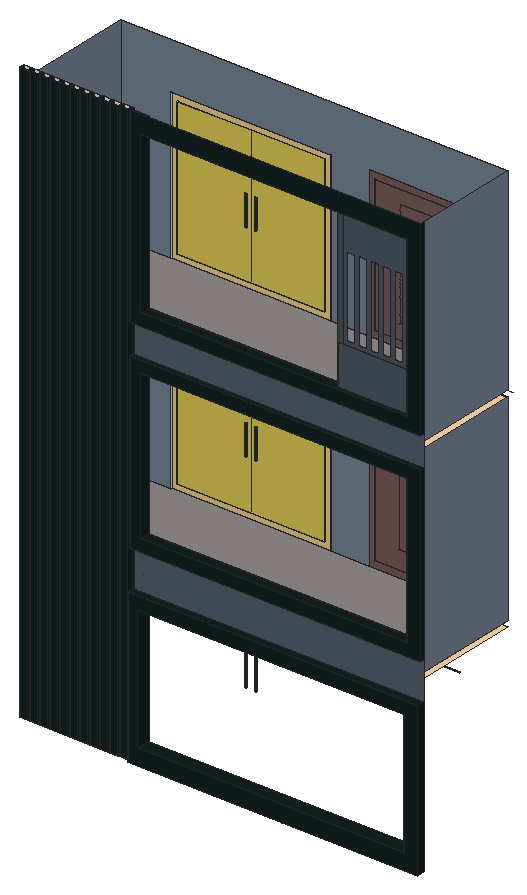
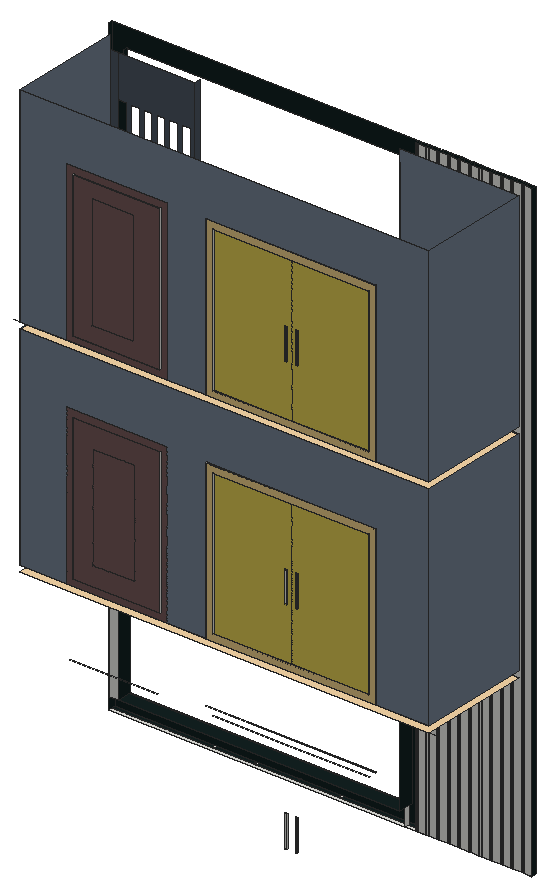
# SketchUp Ruby script. Lengths in millimetres.
U = 1.mm
M = Sketchup.active_model
def pt(a) = Geom::Point3d.new(a.map { |v| v * U })
def face(e, loops, mat)
  f = e.add_face(loops[0].map { |a| pt(a) })
  loops[1..].each { |l| e.add_face(l.map { |a| pt(a) }).erase! }
  f.material = f.back_material = mat if mat
  f
end
# faces: each face lists its corners as indices into pts; further lists are holes
def faces(e, pts, list, mat = nil) = list.each { |f| face(e, (f[0].is_a?(Array) ? f : [f]).map { |l| l.map { |i| pts[i] } }, mat) }
# xy, xz, yz: faces in a plane at the given z, y or x. An outline is a flat list of corners, or four numbers for a rectangle; further outlines are holes
def ring(l) = l.size == 4 ? [[l[0], l[1]], [l[2], l[1]], [l[2], l[3]], [l[0], l[3]]] : l.each_slice(2).to_a
def flat(e, list, mat, &to3) = list.each { |f| face(e, (f[0].is_a?(Array) ? f : [f]).map { |l| ring(l).map { |u, v| to3.(u, v) } }, mat) }
def xy(e, z, list, mat = nil) = flat(e, list, mat) { |x, y| [x, y, z] }
def xz(e, y, list, mat = nil) = flat(e, list, mat) { |x, z| [x, y, z] }
def yz(e, x, list, mat = nil) = flat(e, list, mat) { |y, z| [x, y, z] }
def lines(e, pts, list) = list.each { |a, b| e.add_line(pt(pts[a]), pt(pts[b])) }
# prism: a flat outline (further loops are holes) pulled along v
def prism(e, loops, v, mat = nil)
  f = face(e, loops, mat); d = Geom::Vector3d.new(v.map { |x| x * U })
  f.pushpull(f.normal.samedirection?(d) ? d.length : -d.length)
end
def box(e, o, s, mat = nil) = prism(e, [[o, [o[0] + s[0], o[1], o[2]], [o[0] + s[0], o[1] + s[1], o[2]], [o[0], o[1] + s[1], o[2]]]], [0, 0, s[2]], mat)
def at(x, y, z, deg = 0) = Geom::Transformation.translation(pt([x, y, z])) * Geom::Transformation.rotation(ORIGIN, Z_AXIS, deg.degrees)
def axes(o, x, y, z) = Geom::Transformation.new([*x, 0, *y, 0, *z, 0, *pt(o).to_a, 1])
def part(name) = M.definitions.add(name)
# library, detail: a bought-in or finely detailed component or shape, given as its bounding box
def library(name, o, s) = part(name).tap { |d| box(d.entities, o, s) }
def detail(e, o, s) = box(e.add_group.entities, o, s)
def put(e, d, t, mat = nil) = e.add_instance(d, t).tap { |i| i.material = mat if mat }
def group(e, t, mat = nil) = e.add_group.tap { |g| g.transformation = t; g.material = mat if mat }.entities
root = M.entities
M.materials.add("[0033_NavajoWhite]").color = [249, 217, 169]
M.materials.add("[0078_DarkSlateGray]").color = [19, 33, 33]
M.materials.add("[0099_LightSteelBlue]").color = [113, 126, 142]
M.materials.add("[0110_LightSlateGray]").color = [73, 83, 94]
M.materials.add("[0111_SlateGray]").color = [81, 92, 104]
M.materials.add("[0119_RosyBrown]").color = [114, 87, 87]
M.materials.add("[Checker Plate]").color = [214, 195, 82]
M.materials.add("[Stone Brushed Khaki]").color = [226, 197, 133]
M.materials.add("[Stone Marble]").color = [143, 138, 136]
xy(root,20437.5,[[21124.2,13555.1,21112.3,13555.5,21100.4,13557.1,21088.8,13559.9,21077.5,13564,21066.7,13569.2,21056.6,13575.5,21047.1,13582.8,21038.5,13591.1,21030.8,13600.2,21024,13610.1,21018.4,13620.7,21013.9,13631.8,21010.5,13643.2,21008.4,13655,21007.5,13666.9,21007.9,13678.9,21009.5,13690.8,21012.4,13702.4,21016.4,13713.6,21021.6,13724.4,21027.9,13734.6,21035.2,13744,21043.5,13752.7,21052.7,13760.4,21062.5,13767.1,21073.1,13772.8,21084.2,13777.3,21095.7,13780.6,21107.4,13782.8,21119.4,13783.6,21131.3,13783.3,21143.2,13781.7,21154.8,13778.8,21166,13774.8,21176.8,13769.5,21187,13763.2,21196.4,13755.9,21205.1,13747.6,21212.8,13738.5,21219.5,13728.6,21225.2,13718.1,21229.7,13707,21233.1,13695.5,21235.2,13683.7,21236.1,13671.8,21235.7,13659.8,21234.1,13648,21231.2,13636.4,21227.2,13625.1,21222,13614.3,21215.7,13604.2,21208.3,13594.7,21200.1,13586.1,21190.9,13578.3,21181,13571.6,21170.5,13566,21159.4,13561.4,21147.9,13558.1,21136.1,13556],[24172.2,13555.1,24160.3,13555.5,24148.4,13557.1,24136.8,13559.9,24125.5,13564,24114.7,13569.2,24104.6,13575.5,24095.1,13582.8,24086.5,13591.1,24078.8,13600.2,24072,13610.1,24066.4,13620.7,24061.9,13631.8,24058.5,13643.2,24056.4,13655,24055.5,13666.9,24055.9,13678.9,24057.5,13690.8,24060.4,13702.4,24064.4,13713.6,24069.6,13724.4,24075.9,13734.6,24083.2,13744,24091.5,13752.7,24100.7,13760.4,24110.5,13767.1,24121.1,13772.8,24132.2,13777.3,24143.7,13780.6,24155.4,13782.8,24167.4,13783.6,24179.3,13783.3,24191.2,13781.7,24202.8,13778.8,24214,13774.8,24224.8,13769.5,24235,13763.2,24244.4,13755.9,24253.1,13747.6,24260.8,13738.5,24267.5,13728.6,24273.2,13718.1,24277.7,13707,24281.1,13695.5,24283.2,13683.7,24284.1,13671.8,24283.7,13659.8,24282.1,13648,24279.2,13636.4,24275.2,13625.1,24270,13614.3,24263.7,13604.2,24256.3,13594.7,24248.1,13586.1,24238.9,13578.3,24229,13571.6,24218.5,13566,24207.4,13561.4,24195.9,13558.1,24184.1,13556],[27220.2,13555.1,27208.3,13555.5,27196.4,13557.1,27184.8,13559.9,27173.5,13564,27162.7,13569.2,27152.6,13575.5,27143.1,13582.8,27134.5,13591.1,27126.8,13600.2,27120,13610.1,27114.4,13620.7,27109.9,13631.8,27106.5,13643.2,27104.4,13655,27103.5,13666.9,27103.9,13678.9,27105.5,13690.8,27108.4,13702.4,27112.4,13713.6,27117.6,13724.4,27123.9,13734.6,27131.2,13744,27139.5,13752.7,27148.7,13760.4,27158.5,13767.1,27169.1,13772.8,27180.2,13777.3,27191.7,13780.6,27203.4,13782.8,27215.4,13783.6,27227.3,13783.3,27239.2,13781.7,27250.8,13778.8,27262,13774.8,27272.8,13769.5,27283,13763.2,27292.4,13755.9,27301.1,13747.6,27308.8,13738.5,27315.5,13728.6,27321.2,13718.1,27325.7,13707,27329.1,13695.5,27331.2,13683.7,27332.1,13671.8,27331.7,13659.8,27330.1,13648,27327.2,13636.4,27323.2,13625.1,27318,13614.3,27311.7,13604.2,27304.3,13594.7,27296.1,13586.1,27286.9,13578.3,27277,13571.6,27266.5,13566,27255.4,13561.4,27243.9,13558.1,27232.1,13556],[30268.2,13555.1,30256.3,13555.5,30244.4,13557.1,30232.8,13559.9,30221.5,13564,30210.7,13569.2,30200.6,13575.5,30191.1,13582.8,30182.5,13591.1,30174.8,13600.2,30168,13610.1,30162.4,13620.7,30157.9,13631.8,30154.5,13643.2,30152.4,13655,30151.5,13666.9,30151.9,13678.9,30153.5,13690.8,30156.4,13702.4,30160.4,13713.6,30165.6,13724.4,30171.9,13734.6,30179.2,13744,30187.5,13752.7,30196.7,13760.4,30206.5,13767.1,30217.1,13772.8,30228.2,13777.3,30239.7,13780.6,30251.4,13782.8,30263.4,13783.6,30275.3,13783.3,30287.2,13781.7,30298.8,13778.8,30310,13774.8,30320.8,13769.5,30331,13763.2,30340.4,13755.9,30349.1,13747.6,30356.8,13738.5,30363.5,13728.6,30369.2,13718.1,30373.7,13707,30377.1,13695.5,30379.2,13683.7,30380.1,13671.8,30379.7,13659.8,30378.1,13648,30375.2,13636.4,30371.2,13625.1,30366,13614.3,30359.7,13604.2,30352.3,13594.7,30344.1,13586.1,30334.9,13578.3,30325,13571.6,30314.5,13566,30303.4,13561.4,30291.9,13558.1,30280.1,13556],[7076.1,13804.9,7685.7,14109.7],
  [7685.7,13804.9,7838.1,14109.7],[7838.1,13804.9,8447.7,14109.7],[8447.7,13804.9,8600.1,14109.7],[8600.1,13804.9,9209.7,14109.7],[9209.7,13804.9,9362.1,14109.7],
  [9362.1,13804.9,9971.7,14109.7],[9971.7,13804.9,10124.1,14109.7],[10124.1,13804.9,10733.7,14109.7],[10733.7,13804.9,10886.1,14109.7],[10886.1,13804.9,11495.7,14109.7],
  [11495.7,13804.9,11648.1,14109.7],[11648.1,13804.9,12257.7,14109.7],[12257.7,13804.9,12410.1,14109.7],[12410.1,13804.9,13019.7,14109.7],[13019.7,13804.9,13172.1,14109.7],
  [13172.1,13804.9,13781.7,14109.7],[13781.7,13804.9,13934.1,14109.7],[13934.1,13804.9,14543.7,14109.7],[14543.7,13804.9,14696.1,14109.7],[14696.1,13804.9,15305.7,14109.7],
  [15305.7,13804.9,15458.1,14109.7],[15458.1,13804.9,16220.1,14109.7],[16220.1,13804.9,37556.1,14109.7]])
xy(root,20437.5,[[[15458.1,13527.1,37556.1,13804.9],[24172.2,13555.1,24184.1,13556,24195.9,13558.1,24207.4,13561.4,24218.5,13566,24229,13571.6,24238.9,13578.3,24248.1,13586.1,24256.3,13594.7,24263.7,13604.2,24270,13614.3,24275.2,13625.1,24279.2,13636.4,24282.1,13648,24283.7,13659.8,24284.1,13671.8,24283.2,13683.7,24281.1,13695.5,24277.7,13707,24273.2,13718.1,24267.5,13728.6,24260.8,13738.5,24253.1,13747.6,24244.4,13755.9,24235,13763.2,24224.8,13769.5,24214,13774.8,24202.8,13778.8,24191.2,13781.7,24179.3,13783.3,24167.4,13783.6,24155.4,13782.8,24143.7,13780.6,24132.2,13777.3,24121.1,13772.8,24110.5,13767.1,24100.7,13760.4,24091.5,13752.7,24083.2,13744,24075.9,13734.6,24069.6,13724.4,24064.4,13713.6,24060.4,13702.4,24057.5,13690.8,24055.9,13678.9,24055.5,13666.9,24056.4,13655,24058.5,13643.2,24061.9,13631.8,24066.4,13620.7,24072,13610.1,24078.8,13600.2,24086.5,13591.1,24095.1,13582.8,24104.6,13575.5,24114.7,13569.2,24125.5,13564,24136.8,13559.9,24148.4,13557.1,24160.3,13555.5],[30268.2,13555.1,30280.1,13556,30291.9,13558.1,30303.4,13561.4,30314.5,13566,30325,13571.6,30334.9,13578.3,30344.1,13586.1,30352.3,13594.7,30359.7,13604.2,30366,13614.3,30371.2,13625.1,30375.2,13636.4,30378.1,13648,30379.7,13659.8,30380.1,13671.8,30379.2,13683.7,30377.1,13695.5,30373.7,13707,30369.2,13718.1,30363.5,13728.6,30356.8,13738.5,30349.1,13747.6,30340.4,13755.9,30331,13763.2,30320.8,13769.5,30310,13774.8,30298.8,13778.8,30287.2,13781.7,30275.3,13783.3,30263.4,13783.6,30251.4,13782.8,30239.7,13780.6,30228.2,13777.3,30217.1,13772.8,30206.5,13767.1,30196.7,13760.4,30187.5,13752.7,30179.2,13744,30171.9,13734.6,30165.6,13724.4,30160.4,13713.6,30156.4,13702.4,30153.5,13690.8,30151.9,13678.9,30151.5,13666.9,30152.4,13655,30154.5,13643.2,30157.9,13631.8,30162.4,13620.7,30168,13610.1,30174.8,13600.2,30182.5,13591.1,30191.1,13582.8,30200.6,13575.5,30210.7,13569.2,30221.5,13564,30232.8,13559.9,30244.4,13557.1,30256.3,13555.5],[21124.2,13555.1,21136.1,13556,21147.9,13558.1,21159.4,13561.4,21170.5,13566,21181,13571.6,21190.9,13578.3,21200.1,13586.1,21208.3,13594.7,21215.7,13604.2,21222,13614.3,21227.2,13625.1,21231.2,13636.4,21234.1,13648,21235.7,13659.8,21236.1,13671.8,21235.2,13683.7,21233.1,13695.5,21229.7,13707,21225.2,13718.1,21219.5,13728.6,21212.8,13738.5,21205.1,13747.6,21196.4,13755.9,21187,13763.2,21176.8,13769.5,21166,13774.8,21154.8,13778.8,21143.2,13781.7,21131.3,13783.3,21119.4,13783.6,21107.4,13782.8,21095.7,13780.6,21084.2,13777.3,21073.1,13772.8,21062.5,13767.1,21052.7,13760.4,21043.5,13752.7,21035.2,13744,21027.9,13734.6,21021.6,13724.4,21016.4,13713.6,21012.4,13702.4,21009.5,13690.8,21007.9,13678.9,21007.5,13666.9,21008.4,13655,21010.5,13643.2,21013.9,13631.8,21018.4,13620.7,21024,13610.1,21030.8,13600.2,21038.5,13591.1,21047.1,13582.8,21056.6,13575.5,21066.7,13569.2,21077.5,13564,21088.8,13559.9,21100.4,13557.1,21112.3,13555.5],[27220.2,13555.1,27232.1,13556,27243.9,13558.1,27255.4,13561.4,27266.5,13566,27277,13571.6,27286.9,13578.3,27296.1,13586.1,27304.3,13594.7,27311.7,13604.2,27318,13614.3,27323.2,13625.1,27327.2,13636.4,27330.1,13648,27331.7,13659.8,27332.1,13671.8,27331.2,13683.7,27329.1,13695.5,27325.7,13707,27321.2,13718.1,27315.5,13728.6,27308.8,13738.5,27301.1,13747.6,27292.4,13755.9,27283,13763.2,27272.8,13769.5,27262,13774.8,27250.8,13778.8,27239.2,13781.7,27227.3,13783.3,27215.4,13783.6,27203.4,13782.8,27191.7,13780.6,27180.2,13777.3,27169.1,13772.8,27158.5,13767.1,27148.7,13760.4,27139.5,13752.7,27131.2,13744,27123.9,13734.6,27117.6,13724.4,27112.4,13713.6,27108.4,13702.4,27105.5,13690.8,27103.9,13678.9,27103.5,13666.9,27104.4,13655,27106.5,13643.2,27109.9,13631.8,27114.4,13620.7,27120,13610.1,27126.8,13600.2,27134.5,13591.1,27143.1,13582.8,27152.6,13575.5,27162.7,13569.2,27173.5,13564,27184.8,13559.9,27196.4,13557.1,27208.3,13555.5]]],"[0078_DarkSlateGray]")
xy(root,21656.7,[[16220.1,13527.1,36489.3,14566.9]],"[0078_DarkSlateGray]")
xy(root,22141.2,[[17116.4,22618.7,17268.8,22644.1],[17878.4,22618.7,18030.8,22644.1]])
xy(root,24406.5,[[17116.4,22618.7,17268.8,22644.1],[17878.4,22618.7,18030.8,22644.1]])
xy(root,28873.1,[[11965.2,22644.1,17573.6,22694.9],[17573.6,22644.1,23181.9,22694.9],[27205.2,22644.1,33459.3,22694.9]])
xy(root,29360.8,[[11477.6,22644.1,23669.6,22694.9]])
xy(root,31105.5,[[21294.8,13978.9,21242.7,13988.7,21194.9,14011.7,21154.7,14046.3,21124.8,14090.1,21107.2,14140.2,21103.3,14193.1,21113.1,14245.2,21136.1,14293,21170.7,14333.2,21214.5,14363.1,21264.6,14380.7,21317.5,14384.6,21369.6,14374.8,21417.4,14351.8,21457.6,14317.2,21487.5,14273.4,21505,14223.3,21509,14170.4,21499.2,14118.3,21476.2,14070.5,21441.6,14030.3,21397.8,14000.4,21347.7,13982.8],[26476.4,13978.9,26424.3,13988.7,26376.5,14011.7,26336.3,14046.3,26306.4,14090.1,26288.8,14140.2,26284.9,14193.1,26294.7,14245.2,26317.7,14293,26352.3,14333.2,26396.1,14363.1,26446.2,14380.7,26499.1,14384.6,26551.2,14374.8,26599,14351.8,26639.2,14317.2,26669.1,14273.4,26686.6,14223.3,26690.6,14170.4,26680.8,14118.3,26657.8,14070.5,26623.2,14030.3,26579.4,14000.4,26529.3,13982.8],[31658,13978.9,31605.9,13988.7,31558.1,14011.7,31517.9,14046.3,31488,14090.1,31470.4,14140.2,31466.5,14193.1,31476.3,14245.2,31499.3,14293,31533.9,14333.2,31577.7,14363.1,31627.8,14380.7,31680.7,14384.6,31732.8,14374.8,31780.6,14351.8,31820.8,14317.2,31850.7,14273.4,31868.2,14223.3,31872.2,14170.4,31862.4,14118.3,31839.4,14070.5,31804.8,14030.3,31761,14000.4,31710.9,13982.8]])
xy(root,31105.5,[[[16220.1,13527.1,36489.3,14566.9],[26476.4,13978.9,26529.3,13982.8,26579.4,14000.4,26623.2,14030.3,26657.8,14070.5,26680.8,14118.3,26690.6,14170.4,26686.6,14223.3,26669.1,14273.4,26639.2,14317.2,26599,14351.8,26551.2,14374.8,26499.1,14384.6,26446.2,14380.7,26396.1,14363.1,26352.3,14333.2,26317.7,14293,26294.7,14245.2,26284.9,14193.1,26288.8,14140.2,26306.4,14090.1,26336.3,14046.3,26376.5,14011.7,26424.3,13988.7],[21294.8,13978.9,21347.7,13982.8,21397.8,14000.4,21441.6,14030.3,21476.2,14070.5,21499.2,14118.3,21509,14170.4,21505,14223.3,21487.5,14273.4,21457.6,14317.2,21417.4,14351.8,21369.6,14374.8,21317.5,14384.6,21264.6,14380.7,21214.5,14363.1,21170.7,14333.2,21136.1,14293,21113.1,14245.2,21103.3,14193.1,21107.2,14140.2,21124.8,14090.1,21154.7,14046.3,21194.9,14011.7,21242.7,13988.7],[31658,13978.9,31710.9,13982.8,31761,14000.4,31804.8,14030.3,31839.4,14070.5,31862.4,14118.3,31872.2,14170.4,31868.2,14223.3,31850.7,14273.4,31820.8,14317.2,31780.6,14351.8,31732.8,14374.8,31680.7,14384.6,31627.8,14380.7,31577.7,14363.1,31533.9,14333.2,31499.3,14293,31476.3,14245.2,31466.5,14193.1,31470.4,14140.2,31488,14090.1,31517.9,14046.3,31558.1,14011.7,31605.9,13988.7]]],"[0078_DarkSlateGray]")
xy(root,32019.9,[[15458.1,13527.1,37556.1,14109.7]],"[0078_DarkSlateGray]")
xy(root,33239.1,[[7685.7,14566.9,37098.9,22644.1]],"[0033_NavajoWhite]")
xy(root,33696.3,[[7685.7,14566.9,37098.9,14566.9,37098.9,22644.1,23669.6,22644.1,23669.6,22694.9,11477.6,22694.9,11477.6,22644.1,7685.7,22644.1]],"[Stone Marble]")
xy(root,34184,[[11965.2,22644.1,17573.6,22694.9],[17573.6,22644.1,23181.9,22694.9],[26997.1,22644.1,33251.2,22694.9]])
xy(root,34915.5,[[15458.1,13804.9,37556.1,14109.7]],"[0078_DarkSlateGray]")
xy(root,35829.9,[[16220.1,13804.9,36489.3,14566.9]],"[0078_DarkSlateGray]")
xy(root,37915.5,[[17116.4,22618.7,17268.8,22644.1],[17878.4,22618.7,18030.8,22644.1]])
xy(root,40176.1,[[17116.4,22618.7,17268.8,22644.1],[17878.4,22618.7,18030.8,22644.1]])
xy(root,44570.3,[[11965.2,22644.1,17573.6,22694.9],[17573.6,22644.1,23181.9,22694.9],[26997.1,22644.1,33251.2,22694.9]])
xy(root,45058,[[11477.6,22644.1,23669.6,22694.9]])
xy(root,47107.5,[[20172.2,13993.6,20151,13994.7,20130,13998,20109.4,14003.4,20089.5,14011,20070.5,14020.6,20052.7,14032.1,20036.1,14045.5,20021,14060.5,20007.6,14077,19996,14094.8,19986.3,14113.7,19978.6,14133.5,19973,14154.1,19969.6,14175.1,19968.5,14196.3,19969.5,14217.5,19972.8,14238.6,19978.2,14259.1,19985.8,14279,19995.4,14298,20007,14315.8,20020.3,14332.4,20035.3,14347.5,20051.8,14360.9,20069.6,14372.6,20088.5,14382.3,20108.4,14389.9,20128.9,14395.5,20149.9,14398.9,20171.1,14400,20192.4,14399,20213.4,14395.7,20233.9,14390.3,20253.8,14382.7,20272.8,14373.1,20290.7,14361.6,20307.2,14348.2,20322.3,14333.2,20335.7,14316.7,20347.4,14298.9,20357.1,14280,20364.8,14260.2,20370.3,14239.6,20373.7,14218.6,20374.9,14197.4,20373.8,14176.2,20370.5,14155.1,20365.1,14134.6,20357.5,14114.7,20347.9,14095.7,20336.4,14077.9,20323,14061.3,20308,14046.2,20291.6,14032.8,20273.7,14021.1,20254.8,14011.4,20235,14003.8,20214.5,13998.2,20193.5,13994.8],[23829.8,13993.6,23808.6,13994.7,23787.6,13998,23767,14003.4,23747.1,14011,23728.1,14020.6,23710.3,14032.1,23693.7,14045.5,23678.6,14060.5,23665.2,14077,23653.6,14094.8,23643.9,14113.7,23636.2,14133.5,23630.6,14154.1,23627.2,14175.1,23626.1,14196.3,23627.1,14217.5,23630.4,14238.6,23635.8,14259.1,23643.4,14279,23653,14298,23664.6,14315.8,23677.9,14332.4,23692.9,14347.5,23709.4,14360.9,23727.2,14372.6,23746.1,14382.3,23766,14389.9,23786.5,14395.5,23807.5,14398.9,23828.7,14400,23850,14399,23871,14395.7,23891.5,14390.3,23911.4,14382.7,23930.4,14373.1,23948.3,14361.6,23964.8,14348.2,23979.9,14333.2,23993.3,14316.7,24005,14298.9,24014.7,14280,24022.4,14260.2,24027.9,14239.6,24031.3,14218.6,24032.5,14197.4,24031.4,14176.2,24028.1,14155.1,24022.7,14134.6,24015.1,14114.7,24005.5,14095.7,23994,14077.9,23980.6,14061.3,23965.6,14046.2,23949.2,14032.8,23931.3,14021.1,23912.4,14011.4,23892.6,14003.8,23872.1,13998.2,23851.1,13994.8],[27487.4,13993.6,27466.2,13994.7,27445.2,13998,27424.6,14003.4,27404.7,14011,27385.7,14020.6,27367.9,14032.1,27351.3,14045.5,27336.2,14060.5,27322.8,14077,27311.2,14094.8,27301.5,14113.7,27293.8,14133.5,27288.2,14154.1,27284.8,14175.1,27283.7,14196.3,27284.7,14217.5,27288,14238.6,27293.4,14259.1,27301,14279,27310.6,14298,27322.2,14315.8,27335.5,14332.4,27350.5,14347.5,27367,14360.9,27384.8,14372.6,27403.7,14382.3,27423.6,14389.9,27444.1,14395.5,27465.1,14398.9,27486.3,14400,27507.6,14399,27528.6,14395.7,27549.1,14390.3,27569,14382.7,27588,14373.1,27605.9,14361.6,27622.4,14348.2,27637.5,14333.2,27650.9,14316.7,27662.6,14298.9,27672.3,14280,27680,14260.2,27685.5,14239.6,27688.9,14218.6,27690.1,14197.4,27689,14176.2,27685.7,14155.1,27680.3,14134.6,27672.7,14114.7,27663.1,14095.7,27651.6,14077.9,27638.2,14061.3,27623.2,14046.2,27606.8,14032.8,27588.9,14021.1,27570,14011.4,27550.2,14003.8,27529.7,13998.2,27508.7,13994.8],[31145,13993.6,31123.8,13994.7,31102.8,13998,31082.2,14003.4,31062.3,14011,31043.3,14020.6,31025.5,14032.1,31008.9,14045.5,30993.8,14060.5,30980.4,14077,30968.8,14094.8,30959.1,14113.7,30951.4,14133.5,30945.8,14154.1,30942.4,14175.1,30941.3,14196.3,30942.3,14217.5,30945.6,14238.6,30951,14259.1,30958.6,14279,30968.2,14298,30979.8,14315.8,30993.1,14332.4,31008.1,14347.5,31024.6,14360.9,31042.4,14372.6,31061.3,14382.3,31081.2,14389.9,31101.7,14395.5,31122.7,14398.9,31143.9,14400,31165.2,14399,31186.2,14395.7,31206.7,14390.3,31226.6,14382.7,31245.6,14373.1,31263.5,14361.6,31280,14348.2,31295.1,14333.2,31308.5,14316.7,31320.2,14298.9,31329.9,14280,31337.6,14260.2,31343.1,14239.6,31346.5,14218.6,31347.7,14197.4,31346.6,14176.2,31343.3,14155.1,31337.9,14134.6,31330.3,14114.7,31320.7,14095.7,31309.2,14077.9,31295.8,14061.3,31280.8,14046.2,31264.4,14032.8,31246.5,14021.1,31227.6,14011.4,31207.8,14003.8,31187.3,13998.2,31166.3,13994.8]])
xy(root,47107.5,[[[16220.1,13804.9,36489.3,14566.9],[31145,13993.6,31166.3,13994.8,31187.3,13998.2,31207.8,14003.8,31227.6,14011.4,31246.5,14021.1,31264.4,14032.8,31280.8,14046.2,31295.8,14061.3,31309.2,14077.9,31320.7,14095.7,31330.3,14114.7,31337.9,14134.6,31343.3,14155.1,31346.6,14176.2,31347.7,14197.4,31346.5,14218.6,31343.1,14239.6,31337.6,14260.2,31329.9,14280,31320.2,14298.9,31308.5,14316.7,31295.1,14333.2,31280,14348.2,31263.5,14361.6,31245.6,14373.1,31226.6,14382.7,31206.7,14390.3,31186.2,14395.7,31165.2,14399,31143.9,14400,31122.7,14398.9,31101.7,14395.5,31081.2,14389.9,31061.3,14382.3,31042.4,14372.6,31024.6,14360.9,31008.1,14347.5,30993.1,14332.4,30979.8,14315.8,30968.2,14298,30958.6,14279,30951,14259.1,30945.6,14238.6,30942.3,14217.5,30941.3,14196.3,30942.4,14175.1,30945.8,14154.1,30951.4,14133.5,30959.1,14113.7,30968.8,14094.8,30980.4,14077,30993.8,14060.5,31008.9,14045.5,31025.5,14032.1,31043.3,14020.6,31062.3,14011,31082.2,14003.4,31102.8,13998,31123.8,13994.7],[20172.2,13993.6,20193.5,13994.8,20214.5,13998.2,20235,14003.8,20254.8,14011.4,20273.7,14021.1,20291.6,14032.8,20308,14046.2,20323,14061.3,20336.4,14077.9,20347.9,14095.7,20357.5,14114.7,20365.1,14134.6,20370.5,14155.1,20373.8,14176.2,20374.9,14197.4,20373.7,14218.6,20370.3,14239.6,20364.8,14260.2,20357.1,14280,20347.4,14298.9,20335.7,14316.7,20322.3,14333.2,20307.2,14348.2,20290.7,14361.6,20272.8,14373.1,20253.8,14382.7,20233.9,14390.3,20213.4,14395.7,20192.4,14399,20171.1,14400,20149.9,14398.9,20128.9,14395.5,20108.4,14389.9,20088.5,14382.3,20069.6,14372.6,20051.8,14360.9,20035.3,14347.5,20020.3,14332.4,20007,14315.8,19995.4,14298,19985.8,14279,19978.2,14259.1,19972.8,14238.6,19969.5,14217.5,19968.5,14196.3,19969.6,14175.1,19973,14154.1,19978.6,14133.5,19986.3,14113.7,19996,14094.8,20007.6,14077,20021,14060.5,20036.1,14045.5,20052.7,14032.1,20070.5,14020.6,20089.5,14011,20109.4,14003.4,20130,13998,20151,13994.7],[23829.8,13993.6,23851.1,13994.8,23872.1,13998.2,23892.6,14003.8,23912.4,14011.4,23931.3,14021.1,23949.2,14032.8,23965.6,14046.2,23980.6,14061.3,23994,14077.9,24005.5,14095.7,24015.1,14114.7,24022.7,14134.6,24028.1,14155.1,24031.4,14176.2,24032.5,14197.4,24031.3,14218.6,24027.9,14239.6,24022.4,14260.2,24014.7,14280,24005,14298.9,23993.3,14316.7,23979.9,14333.2,23964.8,14348.2,23948.3,14361.6,23930.4,14373.1,23911.4,14382.7,23891.5,14390.3,23871,14395.7,23850,14399,23828.7,14400,23807.5,14398.9,23786.5,14395.5,23766,14389.9,23746.1,14382.3,23727.2,14372.6,23709.4,14360.9,23692.9,14347.5,23677.9,14332.4,23664.6,14315.8,23653,14298,23643.4,14279,23635.8,14259.1,23630.4,14238.6,23627.1,14217.5,23626.1,14196.3,23627.2,14175.1,23630.6,14154.1,23636.2,14133.5,23643.9,14113.7,23653.6,14094.8,23665.2,14077,23678.6,14060.5,23693.7,14045.5,23710.3,14032.1,23728.1,14020.6,23747.1,14011,23767,14003.4,23787.6,13998,23808.6,13994.7],[27487.4,13993.6,27508.7,13994.8,27529.7,13998.2,27550.2,14003.8,27570,14011.4,27588.9,14021.1,27606.8,14032.8,27623.2,14046.2,27638.2,14061.3,27651.6,14077.9,27663.1,14095.7,27672.7,14114.7,27680.3,14134.6,27685.7,14155.1,27689,14176.2,27690.1,14197.4,27688.9,14218.6,27685.5,14239.6,27680,14260.2,27672.3,14280,27662.6,14298.9,27650.9,14316.7,27637.5,14333.2,27622.4,14348.2,27605.9,14361.6,27588,14373.1,27569,14382.7,27549.1,14390.3,27528.6,14395.7,27507.6,14399,27486.3,14400,27465.1,14398.9,27444.1,14395.5,27423.6,14389.9,27403.7,14382.3,27384.8,14372.6,27367,14360.9,27350.5,14347.5,27335.5,14332.4,27322.2,14315.8,27310.6,14298,27301,14279,27293.4,14259.1,27288,14238.6,27284.7,14217.5,27283.7,14196.3,27284.8,14175.1,27288.2,14154.1,27293.8,14133.5,27301.5,14113.7,27311.2,14094.8,27322.8,14077,27336.2,14060.5,27351.3,14045.5,27367.9,14032.1,27385.7,14020.6,27404.7,14011,27424.6,14003.4,27445.2,13998,27466.2,13994.7]]],"[0078_DarkSlateGray]")
xy(root,48021.9,[[15458.1,13804.9,37556.1,14109.7]],"[0078_DarkSlateGray]")
xy(root,48936.3,[[7685.7,14566.9,37098.9,22644.1]],"[0033_NavajoWhite]")
xy(root,49393.5,[[7685.7,14566.9,37098.9,14566.9,37098.9,22644.1,23669.6,22644.1,23669.6,22694.9,11477.6,22694.9,11477.6,22644.1,7685.7,22644.1]],"[Stone Marble]")
xy(root,49881.2,[[11965.2,22644.1,17573.6,22694.9],[17573.6,22644.1,23181.9,22694.9],[26997.1,22644.1,33251.2,22694.9]])
xy(root,50307.9,[[15458.1,13804.9,37556.1,14109.7]],"[0078_DarkSlateGray]")
xy(root,51222.3,[[31002.9,14109.7,36489.3,14566.9]])
xy(root,51222.3,[[16220.1,13804.9,36489.3,13804.9,36489.3,14109.7,31002.9,14109.7,31002.9,14566.9,16220.1,14566.9]],"[0078_DarkSlateGray]")
xy(root,53561.9,[[17116.4,22593.3,17268.8,22644.1],[17878.4,22593.3,18030.8,22644.1]])
xz(root,13527.1,[[[15458.1,20437.5,37556.1,32019.9],[16220.1,21656.7,36489.3,31105.5]]],"[0078_DarkSlateGray]")
xz(root,13804.9,[[7076.1,20437.5,7685.7,64785.9],[7838.1,20437.5,8447.7,64785.9],[8600.1,20437.5,9209.7,64785.9],[9362.1,20437.5,9971.7,64785.9],[10124.1,20437.5,10733.7,64785.9],
  [10886.1,20437.5,11495.7,64785.9],[11648.1,20437.5,12257.7,64785.9],[12410.1,20437.5,13019.7,64785.9],[13172.1,20437.5,13781.7,64785.9],[13934.1,20437.5,14543.7,64785.9],
  [14696.1,20437.5,15305.7,64785.9],[[15458.1,34915.5,37556.1,48021.9],[16220.1,35829.9,36489.3,47107.5]],[[15458.1,50307.9,37556.1,64785.9],[16220.1,51222.3,36489.3,63414.3]]],"[0078_DarkSlateGray]")
xz(root,14109.7,[[7076.1,20437.5,7685.7,64785.9],[7685.7,20437.5,7838.1,64785.9],[7838.1,20437.5,8447.7,64785.9],[8447.7,20437.5,8600.1,64785.9],[8600.1,20437.5,9209.7,64785.9],
  [9209.7,20437.5,9362.1,64785.9],[9362.1,20437.5,9971.7,64785.9],[9971.7,20437.5,10124.1,64785.9],[10124.1,20437.5,10733.7,64785.9],[10733.7,20437.5,10886.1,64785.9],
  [10886.1,20437.5,11495.7,64785.9],[11495.7,20437.5,11648.1,64785.9],[11648.1,20437.5,12257.7,64785.9],[12257.7,20437.5,12410.1,64785.9],[12410.1,20437.5,13019.7,64785.9],
  [13019.7,20437.5,13172.1,64785.9],[13172.1,20437.5,13781.7,64785.9],[13781.7,20437.5,13934.1,64785.9],[13934.1,20437.5,14543.7,64785.9],[14543.7,20437.5,14696.1,64785.9],
  [14696.1,20437.5,15305.7,64785.9]])
xz(root,14109.7,[[15305.7,20437.5,15458.1,64785.9]],"[0078_DarkSlateGray]")
xz(root,14109.7,[[31002.9,51222.3,36489.3,54270.3]],"[0110_LightSlateGray]")
xz(root,14109.7,[[15458.1,32019.9,37556.1,34915.5],[15458.1,48021.9,37556.1,50307.9]],"[0111_SlateGray]")
xz(root,14566.9,[[36489.3,21656.7,37098.9,31105.5],[16220.1,31105.5,37098.9,31410.3],[16220.1,31410.3,37098.9,33239.1],[36489.3,33696.3,37098.9,47107.5],[16220.1,47107.5,37098.9,48936.3]])
xz(root,14566.9,[[7685.7,33696.3,7685.7,48936.3,16220.1,48936.3,16220.1,35829.9,36489.3,35829.9,36489.3,33696.3],[7685.7,49393.5,7685.7,64328.7,16220.1,64328.7,16220.1,51222.3,36489.3,51222.3,36489.3,49393.5]],"[0099_LightSteelBlue]")
xz(root,14566.9,[[36489.3,49393.5,37098.9,63414.3],[[31002.9,51222.3,31002.9,63414.3,36489.3,63414.3,36489.3,60366.3,35879.7,60366.3,35879.7,54270.3,36489.3,54270.3,36489.3,51222.3],[33136.5,54270.3,33746.1,60366.3],[34965.3,54270.3,35574.9,60366.3],[32222.1,54270.3,32831.7,60366.3],[34050.9,54270.3,34660.5,60366.3],[31307.7,54270.3,31917.3,60366.3]]],"[0110_LightSlateGray]")
xz(root,22593.3,[[17116.4,53561.9,17268.8,55822.5],[17878.4,53561.9,18030.8,55822.5]])
xz(root,22618.7,[[17116.4,22141.2,17268.8,24406.5],[17878.4,22141.2,18030.8,24406.5],[17116.4,37915.5,17268.8,40176.1],[17878.4,37915.5,18030.8,40176.1]])
xz(root,22644.1,[[17116.4,53561.9,17268.8,55822.5],[17878.4,53561.9,18030.8,55822.5]])
xz(root,22644.1,[[7685.7,33696.3,11477.6,33696.3,11477.6,45058,23669.6,45058,23669.6,33696.3,26509.4,33696.3,26509.4,45058,33738.9,45058,33738.9,33696.3,37098.9,33696.3,37098.9,48936.3,7685.7,48936.3],[7685.7,49393.5,11477.6,49393.5,11477.6,60755.2,23669.6,60755.2,23669.6,49393.5,26509.4,49393.5,26509.4,60755.2,33738.9,60755.2,33738.9,49393.5,37098.9,49393.5,37098.9,64328.7,7685.7,64328.7]],"[0099_LightSteelBlue]")
xz(root,22644.1,[[[26509.4,33696.3,33738.9,45058],[26997.1,34184,33251.2,44570.3]],[[26509.4,49393.5,33738.9,60755.2],[26997.1,49881.2,33251.2,60267.5]]],"[0119_RosyBrown]")
xz(root,22644.1,[[[11965.2,34184,17573.6,44570.3],[17116.4,37915.5,17268.8,40176.1]],[[17573.6,34184,23181.9,44570.3],[17878.4,37915.5,18030.8,40176.1]],[[11965.2,49881.2,17573.6,60267.5],[17116.4,53561.9,17268.8,55822.5]],[[17573.6,49881.2,23181.9,60267.5],[17878.4,53561.9,18030.8,55822.5]]],"[Checker Plate]")
xz(root,22694.9,[[[26997.1,34184,33251.2,44570.3],[28810.6,35542.6,31833.2,43103.9]],[28810.6,35542.6,31833.2,43103.9],[[26997.1,49881.2,33251.2,60267.5],[28856.8,51003.6,31892.1,59222.1]],[28856.8,51003.6,31892.1,59222.1]],"[0119_RosyBrown]")
xz(root,22694.9,[[[11477.6,33696.3,23669.6,45058],[11965.2,34184,23181.9,44570.3]],[[11477.6,49393.5,23669.6,60755.2],[11965.2,49881.2,23181.9,60267.5]]],"[Stone Brushed Khaki]")
yz(root,7076.1,[[13804.9,20437.5,14109.7,64785.9]],"[0078_DarkSlateGray]")
yz(root,7685.7,[[13804.9,20437.5,14109.7,64785.9]],"[0078_DarkSlateGray]")
yz(root,7685.7,[[14566.9,33696.3,22644.1,48936.3],[14566.9,49393.5,22644.1,64328.7]],"[0099_LightSteelBlue]")
yz(root,7838.1,[[13804.9,20437.5,14109.7,64785.9]],"[0078_DarkSlateGray]")
yz(root,8447.7,[[13804.9,20437.5,14109.7,64785.9]],"[0078_DarkSlateGray]")
yz(root,8600.1,[[13804.9,20437.5,14109.7,64785.9]],"[0078_DarkSlateGray]")
yz(root,9209.7,[[13804.9,20437.5,14109.7,64785.9]],"[0078_DarkSlateGray]")
yz(root,9362.1,[[13804.9,20437.5,14109.7,64785.9]],"[0078_DarkSlateGray]")
yz(root,9971.7,[[13804.9,20437.5,14109.7,64785.9]],"[0078_DarkSlateGray]")
yz(root,10124.1,[[13804.9,20437.5,14109.7,64785.9]],"[0078_DarkSlateGray]")
yz(root,10733.7,[[13804.9,20437.5,14109.7,64785.9]],"[0078_DarkSlateGray]")
yz(root,10886.1,[[13804.9,20437.5,14109.7,64785.9]],"[0078_DarkSlateGray]")
yz(root,11477.6,[[22644.1,33696.3,22694.9,45058],[22644.1,49393.5,22694.9,60755.2]])
yz(root,11495.7,[[13804.9,20437.5,14109.7,64785.9]],"[0078_DarkSlateGray]")
yz(root,11648.1,[[13804.9,20437.5,14109.7,64785.9]],"[0078_DarkSlateGray]")
yz(root,11965.2,[[22644.1,34184,22694.9,44570.3],[22644.1,49881.2,22694.9,60267.5]])
yz(root,12257.7,[[13804.9,20437.5,14109.7,64785.9]],"[0078_DarkSlateGray]")
yz(root,12410.1,[[13804.9,20437.5,14109.7,64785.9]],"[0078_DarkSlateGray]")
yz(root,13019.7,[[13804.9,20437.5,14109.7,64785.9]],"[0078_DarkSlateGray]")
yz(root,13172.1,[[13804.9,20437.5,14109.7,64785.9]],"[0078_DarkSlateGray]")
yz(root,13781.7,[[13804.9,20437.5,14109.7,64785.9]],"[0078_DarkSlateGray]")
yz(root,13934.1,[[13804.9,20437.5,14109.7,64785.9]],"[0078_DarkSlateGray]")
yz(root,14543.7,[[13804.9,20437.5,14109.7,64785.9]],"[0078_DarkSlateGray]")
yz(root,14696.1,[[13804.9,20437.5,14109.7,64785.9]],"[0078_DarkSlateGray]")
yz(root,15305.7,[[13804.9,20437.5,14109.7,64785.9]],"[0078_DarkSlateGray]")
yz(root,15458.1,[[13527.1,20437.5,14109.7,32019.9],[13804.9,34915.5,14109.7,48021.9],[13804.9,50307.9,14109.7,64785.9]],"[0078_DarkSlateGray]")
yz(root,16220.1,[[13804.9,20437.5,14109.7,21656.7]])
yz(root,16220.1,[[13527.1,21656.7,14566.9,31105.5],[13804.9,35829.9,14566.9,47107.5],[13804.9,51222.3,14566.9,63414.3]],"[0078_DarkSlateGray]")
yz(root,17116.4,[[22618.7,22141.2,22644.1,24406.5],[22618.7,37915.5,22644.1,40176.1],[22593.3,53561.9,22644.1,55822.5]])
yz(root,17268.8,[[22618.7,22141.2,22644.1,24406.5],[22618.7,37915.5,22644.1,40176.1],[22593.3,53561.9,22644.1,55822.5]])
yz(root,17878.4,[[22618.7,22141.2,22644.1,24406.5],[22618.7,37915.5,22644.1,40176.1],[22593.3,53561.9,22644.1,55822.5]])
yz(root,18030.8,[[22618.7,22141.2,22644.1,24406.5],[22618.7,37915.5,22644.1,40176.1],[22593.3,53561.9,22644.1,55822.5]])
yz(root,23181.9,[[22644.1,34184,22694.9,44570.3],[22644.1,49881.2,22694.9,60267.5]])
yz(root,23669.6,[[22644.1,33696.3,22694.9,45058],[22644.1,49393.5,22694.9,60755.2]])
yz(root,26997.1,[[22644.1,34184,22694.9,44570.3],[22644.1,49881.2,22694.9,60267.5]])
yz(root,31002.9,[[14109.7,51222.3,14566.9,63414.3]],"[0110_LightSlateGray]")
yz(root,33251.2,[[22644.1,34184,22694.9,44570.3],[22644.1,49881.2,22694.9,60267.5]])
yz(root,36489.3,[[14109.7,51222.3,14566.9,54270.3]])
yz(root,36489.3,[[13527.1,21656.7,14566.9,31105.5],[13804.9,35829.9,14566.9,47107.5],[13804.9,51222.3,13804.9,63414.3,14109.7,63414.3,14109.7,60366.3,14566.9,60366.3,14566.9,54270.3,14109.7,54270.3,14109.7,51222.3]],"[0078_DarkSlateGray]")
yz(root,37098.9,[[14566.9,33696.3,22644.1,48936.3],[14566.9,49393.5,22644.1,64328.7]],"[0099_LightSteelBlue]")
yz(root,37556.1,[[13527.1,20437.5,14109.7,32019.9],[13804.9,34915.5,14109.7,48021.9],[13804.9,50307.9,14109.7,64785.9]],"[0078_DarkSlateGray]")
p = [[7076.1,22644.1,33239.1],[7685.7,22644.1,33239.1],[16220.1,14566.9,33239.1],[16220.1,14109.7,33239.1],[37098.9,14109.7,49393.5],[37098.9,14566.9,49393.5],
  [37556.1,22644.1,49393.5],[37098.9,22644.1,49393.5],[36489.3,14109.7,50307.9],[36489.3,14566.9,50307.9],[37098.9,14566.9,47107.5],[37098.9,14109.7,47107.5],
  [36489.3,14566.9,35525.1],[36489.3,14109.7,35525.1],[16220.1,14566.9,31410.3],[16220.1,14109.7,31410.3],[37098.9,14566.9,31410.3],[37098.9,14109.7,31410.3],
  [37098.9,14566.9,21656.7],[37098.9,14109.7,21656.7]]
lines(root,p,[[0,1],[2,3],[4,5],[6,7],[8,9],[10,11],[12,13],[14,15],[16,17],[18,19]])
